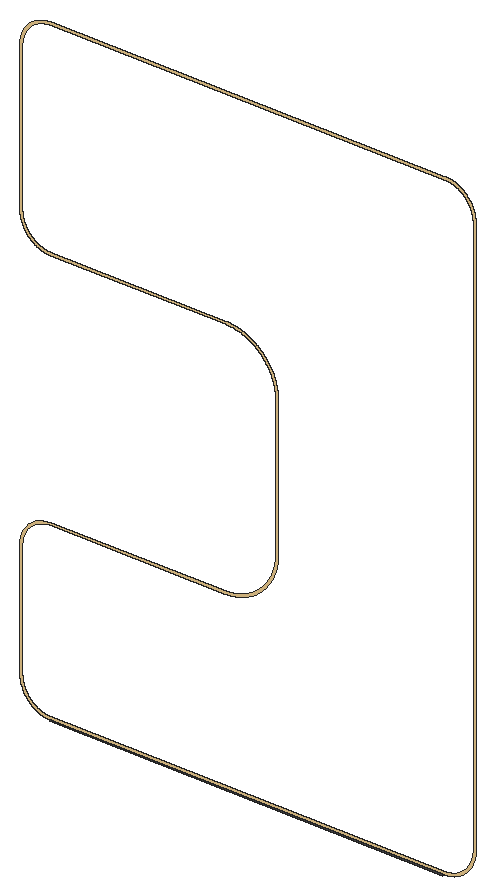
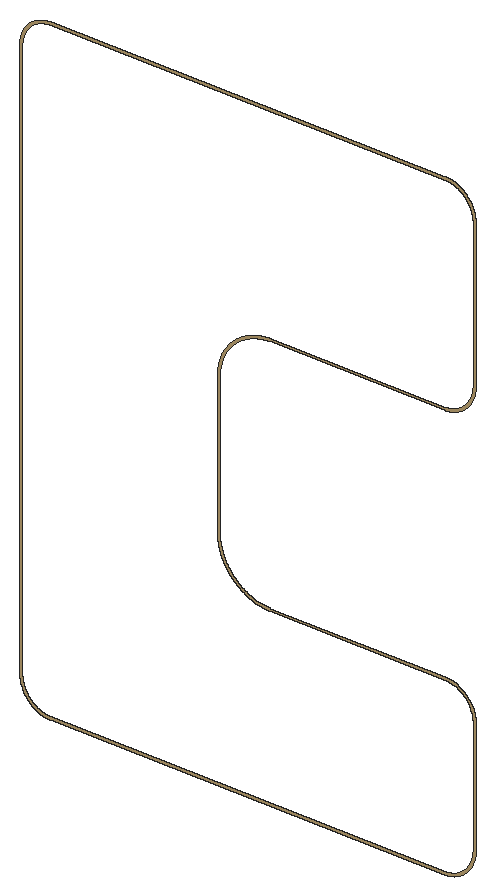
# SketchUp Ruby script. Lengths in inches.
U = 1.inch
M = Sketchup.active_model
def pt(a) = Geom::Point3d.new(a.map { |v| v * U })
def face(e, loops, mat)
  f = e.add_face(loops[0].map { |a| pt(a) })
  loops[1..].each { |l| e.add_face(l.map { |a| pt(a) }).erase! }
  f.material = f.back_material = mat if mat
  f
end
# faces: each face lists its corners as indices into pts; further lists are holes
def faces(e, pts, list, mat = nil) = list.each { |f| face(e, (f[0].is_a?(Array) ? f : [f]).map { |l| l.map { |i| pts[i] } }, mat) }
# xy, xz, yz: faces in a plane at the given z, y or x. An outline is a flat list of corners, or four numbers for a rectangle; further outlines are holes
def ring(l) = l.size == 4 ? [[l[0], l[1]], [l[2], l[1]], [l[2], l[3]], [l[0], l[3]]] : l.each_slice(2).to_a
def flat(e, list, mat, &to3) = list.each { |f| face(e, (f[0].is_a?(Array) ? f : [f]).map { |l| ring(l).map { |u, v| to3.(u, v) } }, mat) }
def xy(e, z, list, mat = nil) = flat(e, list, mat) { |x, y| [x, y, z] }
def xz(e, y, list, mat = nil) = flat(e, list, mat) { |x, z| [x, y, z] }
def yz(e, x, list, mat = nil) = flat(e, list, mat) { |y, z| [x, y, z] }
def lines(e, pts, list) = list.each { |a, b| e.add_line(pt(pts[a]), pt(pts[b])) }
# prism: a flat outline (further loops are holes) pulled along v
def prism(e, loops, v, mat = nil)
  f = face(e, loops, mat); d = Geom::Vector3d.new(v.map { |x| x * U })
  f.pushpull(f.normal.samedirection?(d) ? d.length : -d.length)
end
def box(e, o, s, mat = nil) = prism(e, [[o, [o[0] + s[0], o[1], o[2]], [o[0] + s[0], o[1] + s[1], o[2]], [o[0], o[1] + s[1], o[2]]]], [0, 0, s[2]], mat)
def at(x, y, z, deg = 0) = Geom::Transformation.translation(pt([x, y, z])) * Geom::Transformation.rotation(ORIGIN, Z_AXIS, deg.degrees)
def axes(o, x, y, z) = Geom::Transformation.new([*x, 0, *y, 0, *z, 0, *pt(o).to_a, 1])
def part(name) = M.definitions.add(name)
# library, detail: a bought-in or finely detailed component or shape, given as its bounding box
def library(name, o, s) = part(name).tap { |d| box(d.entities, o, s) }
def detail(e, o, s) = box(e.add_group.entities, o, s)
def put(e, d, t, mat = nil) = e.add_instance(d, t).tap { |i| i.material = mat if mat }
def group(e, t, mat = nil) = e.add_group.tap { |g| g.transformation = t; g.material = mat if mat }.entities
root = M.entities
M.materials.add("1432 AP 8245 TAR ROAD").color = [71, 72, 75]
M.materials.add("Outer Light").color = [251, 217, 152]
xy(root,171.29,[[279,95.37,537,96.87]],"1432 AP 8245 TAR ROAD")
xz(root,96.87,[[[278.68,171.29,278.52,171.3,278.36,171.3,278.2,171.31,278.03,171.31,277.875,171.32,277.71,171.33,277.55,171.34,277.39,171.36,277.07,171.38,276.75,171.42,276.59,171.43,276.27,171.47,276.11,171.5,275.79,171.54,275.63,171.57,275.48,171.6,275.32,171.625,275.16,171.66,275,171.6875,274.84,171.72,274.69,171.75,274.53,171.79,274.37,171.82,274.21,171.86,274.06,171.9,273.9,171.9375,273.75,171.98,273.59,172.02,273.44,172.0625,273.28,172.11,273.125,172.15,272.97,172.2,272.67,172.3,272.51,172.35,272.06,172.5,271.9,172.56,271.75,172.62,271.6,172.67,271.15,172.85,271.01,172.91,270.86,172.98,270.71,173.04,270.5625,173.11,270.42,173.18,270.27,173.24,270.125,173.3125,269.98,173.38,269.84,173.45,269.69,173.53,269.41,173.67,269.27,173.75,268.98,173.91,268.56,174.15,268.43,174.23,268.29,174.3125,268.15,174.4,268.02,174.48,267.88,174.57,267.75,174.66,267.61,174.75,267.48,174.84,267.34,174.93,267.08,175.11,266.95,175.21,266.82,175.3,266.69,175.4,266.5625,175.5,266.44,175.59,266.18,175.79,266.06,175.89,265.93,176,265.81,176.1,265.6875,176.2,265.5625,176.31,265.44,176.41,265.08,176.74,264.97,176.85,264.73,177.07,264.39,177.41,264.28,177.53,264.17,177.64,264.06,177.76,263.95,177.875,263.84,178,263.73,178.11,263.62,178.24,263.52,178.36,263.41,178.48,263.31,178.6,263.2,178.72,263.1,178.85,263,178.97,262.7,179.36,262.61,179.48,262.51,179.61,262.42,179.74,262.32,179.875,262.23,180,262.14,180.14,262.04,180.27,261.95,180.4,261.87,180.54,261.78,180.67,261.69,180.81,261.61,180.94,261.52,181.08,261.4375,181.22,261.35,181.36,261.11,181.78,261.04,181.92,260.88,182.2,260.81,182.34,260.73,182.49,260.59,182.77,260.52,182.92,260.45,183.0625,260.38,183.21,260.32,183.36,260.25,183.5,260.1875,183.65,260.12,183.8,259.82,184.55,259.77,184.7,259.71,184.85,259.61,185.15,259.55,185.3,259.5,185.46,259.45,185.61,259.41,185.76,259.36,185.92,259.3125,186.07,259.27,186.23,259.23,186.38,259.18,186.54,259.14,186.69,259.1,186.85,259.07,187.01,259.03,187.16,258.99,187.32,258.96,187.48,258.93,187.63,258.89,187.79,258.83,188.11,258.81,188.27,258.75,188.59,258.73,188.74,258.7,188.9,258.68,189.0625,258.66,189.22,258.64,189.38,258.61,189.7,258.59,189.86,258.58,190.02,258.5625,190.18,258.55,190.34,258.54,190.5,258.53,190.67,258.52,190.83,258.52,190.99,258.51,191.15,258.51,191.31,258.5,191.47,258.5,266.79,258.68,269.47,259.2,272.1,260.06,274.64,261.25,277.04,262.74,279.27,264.5,281.29,266.52,283.06,268.75,284.55,271.15,285.73,273.69,286.59,276.32,287.12,279,287.29,393.4375,287.29,393.875,287.3,394.32,287.32,394.75,287.34,395.19,287.36,395.63,287.4,396.07,287.43,396.5,287.48,396.9375,287.52,397.37,287.58,397.81,287.64,398.24,287.7,398.67,287.78,399.1,287.85,399.54,287.9375,399.97,288.02,400.39,288.12,401.25,288.32,401.67,288.43,402.51,288.67,403.35,288.93,403.77,289.07,404.18,289.21,404.59,289.36,405.01,289.52,405.41,289.68,405.82,289.84,406.22,290.01,406.625,290.1875,407.03,290.37,407.42,290.56,407.82,290.75,408.21,290.94,408.6,291.14,408.98,291.35,409.37,291.5625,409.75,291.78,410.13,292,410.5,292.23,410.875,292.46,411.25,292.7,411.61,292.9375,411.97,293.18,412.33,293.43,412.69,293.69,413.39,294.21,413.74,294.48,414.76,295.32,415.42,295.9,415.74,296.19,416.06,296.49,416.375,296.8,416.6875,297.1,417,297.42,417.3,297.73,417.6,298.05,417.9,298.375,418.1875,298.7,418.47,299.04,418.76,299.37,419.03,299.71,419.31,300.05,419.58,300.4,420.1,301.1,420.36,301.46,420.61,301.82,420.85,302.18,421.1,302.55,421.33,302.92,421.5625,303.29,421.79,303.66,422.23,304.42,422.44,304.81,422.65,305.19,422.85,305.58,423.05,305.98,423.24,306.37,423.78,307.57,423.95,307.97,424.12,308.38,424.27,308.79,424.43,309.2,424.58,309.61,424.72,310.02,424.86,310.44,425.12,311.28,425.36,312.12,425.47,312.55,425.57,312.97,425.77,313.83,425.86,314.26,425.9375,314.6875,426.02,315.12,426.09,315.55,426.15,315.99,426.27,316.85,426.32,317.29,426.36,317.73,426.4,318.16,426.43,318.6,426.49,319.92,426.5,320.35,426.5,411.23,426.49,411.67,426.45,412.55,426.43,412.98,426.4,413.42,426.36,413.86,426.32,414.29,426.27,414.73,426.21,415.16,426.15,415.6,426.09,416.03,426.02,416.47,425.9375,416.9,425.86,417.33,425.77,417.76,425.67,418.19,425.57,418.61,425.47,419.04,425.36,419.46,425.24,419.89,425.12,420.31,424.99,420.73,424.86,421.14,424.72,421.56,424.58,421.97,424.43,422.39,424.27,422.8,424.12,423.21,423.95,423.61,423.78,424.02,423.42,424.82,423.24,425.21,423.05,425.61,422.65,426.39,422.44,426.78,422.23,427.16,421.79,427.92,421.5625,428.3,421.33,428.67,421.1,429.04,420.85,429.4,420.61,429.77,420.36,430.125,420.1,430.48,419.84,430.84,419.58,431.1875,419.31,431.53,419.03,431.875,418.76,432.21,418.47,432.55,418.1875,432.88,417.9,433.21,417,434.17,416.375,434.79,416.06,435.09,415.74,435.39,415.42,435.6875,415.09,435.98,414.76,436.27,414.08,436.83,413.74,437.1,413.39,437.37,412.69,437.89,412.33,438.15,411.61,438.65,411.25,438.89,410.5,439.36,410.13,439.58,409.37,440.02,408.98,440.23,408.6,440.4375,408.21,440.64,407.82,440.84,407.42,441.03,407.03,441.21,406.625,441.4,406.22,441.57,405.82,441.74,405.41,441.91,405.01,442.07,404.59,442.22,404.18,442.37,403.77,442.51,402.93,442.79,401.67,443.15,401.25,443.26,400.82,443.37,400.39,443.47,399.97,443.56,399.54,443.65,399.1,443.73,398.67,443.81,397.81,443.95,397.37,444.01,396.9375,444.06,396.5,444.11,396.07,444.15,395.63,444.1875,395.19,444.22,394.75,444.25,394.32,444.27,393.875,444.28,393.4375,444.29,278.68,444.29,278.52,444.3,278.36,444.3,278.2,444.31,278.03,444.31,277.875,444.32,277.71,444.33,277.55,444.34,277.39,444.36,277.07,444.38,276.75,444.42,276.59,444.43,276.27,444.47,276.11,444.5,275.79,444.54,275.63,444.57,275.48,444.6,275.32,444.625,275.16,444.66,275,444.6875,274.84,444.72,274.69,444.75,274.53,444.79,274.37,444.82,274.21,444.86,274.06,444.9,273.9,444.9375,273.75,444.98,273.59,445.02,273.44,445.0625,273.28,445.11,273.125,445.15,272.97,445.2,272.67,445.3,272.51,445.35,272.06,445.5,271.9,445.56,271.75,445.62,271.6,445.67,271.15,445.85,271.01,445.91,270.86,445.98,270.71,446.04,270.5625,446.11,270.42,446.18,270.27,446.24,270.125,446.3125,269.98,446.38,269.84,446.45,269.69,446.53,269.41,446.67,269.27,446.75,268.98,446.91,268.56,447.15,268.43,447.23,268.29,447.3125,268.15,447.4,268.02,447.48,267.88,447.57,267.75,447.66,267.61,447.75,267.48,447.84,267.34,447.93,267.08,448.11,266.95,448.21,266.82,448.3,266.69,448.4,266.5625,448.5,266.44,448.59,266.18,448.79,266.06,448.89,265.93,449,265.81,449.1,265.6875,449.2,265.5625,449.31,265.44,449.41,265.08,449.74,264.97,449.85,264.73,450.07,264.39,450.41,264.28,450.53,264.17,450.64,264.06,450.76,263.95,450.875,263.84,451,263.73,451.11,263.62,451.24,263.52,451.36,263.41,451.48,263.31,451.6,263.2,451.72,263.1,451.85,263,451.97,262.7,452.36,262.61,452.48,262.51,452.61,262.42,452.74,262.32,452.875,262.23,453,262.14,453.14,262.04,453.27,261.95,453.4,261.87,453.54,261.78,453.67,261.69,453.81,261.61,453.94,261.52,454.08,261.4375,454.22,261.35,454.36,261.11,454.78,261.04,454.92,260.88,455.2,260.81,455.34,260.73,455.49,260.59,455.77,260.52,455.92,260.45,456.0625,260.38,456.21,260.32,456.36,260.25,456.5,260.1875,456.65,260.12,456.8,259.82,457.55,259.77,457.7,259.71,457.85,259.61,458.15,259.55,458.3,259.5,458.46,259.45,458.61,259.41,458.76,259.36,458.92,259.3125,459.07,259.27,459.23,259.23,459.38,259.18,459.54,259.14,459.69,259.1,459.85,259.07,460.01,259.03,460.16,258.99,460.32,258.96,460.48,258.93,460.63,258.89,460.79,258.83,461.11,258.81,461.27,258.75,461.59,258.73,461.74,258.7,461.9,258.68,462.0625,258.66,462.22,258.64,462.38,258.61,462.7,258.59,462.86,258.58,463.02,258.5625,463.18,258.55,463.34,258.54,463.5,258.53,463.67,258.52,463.83,258.52,463.99,258.51,464.15,258.51,464.31,258.5,464.47,258.5,561.11,258.51,561.28,258.51,561.4375,258.52,561.6,258.52,561.76,258.55,562.24,258.5625,562.4,258.58,562.5625,258.59,562.72,258.61,562.88,258.64,563.2,258.7,563.68,258.73,563.84,258.75,564,258.81,564.32,258.83,564.48,258.86,564.63,258.89,564.79,258.93,564.95,258.96,565.11,258.99,565.26,259.07,565.58,259.1,565.73,259.18,566.05,259.23,566.2,259.27,566.36,259.3125,566.51,259.36,566.67,259.41,566.82,259.45,566.97,259.55,567.28,259.61,567.43,259.66,567.58,259.71,567.74,259.77,567.89,259.82,568.04,259.88,568.1875,259.94,568.34,260.12,568.79,260.1875,568.93,260.25,569.08,260.32,569.23,260.38,569.375,260.45,569.52,260.52,569.67,260.59,569.8125,260.66,569.96,260.73,570.1,260.81,570.24,260.88,570.38,260.96,570.53,261.04,570.67,261.11,570.81,261.35,571.23,261.4375,571.37,261.52,571.5,261.61,571.64,261.69,571.78,261.78,571.91,261.87,572.05,261.95,572.18,262.04,572.31,262.14,572.45,262.32,572.71,262.42,572.84,262.51,572.97,262.61,573.1,262.7,573.23,262.8,573.36,262.9,573.48,263,573.61,263.1,573.73,263.2,573.86,263.31,573.98,263.41,574.11,263.52,574.23,263.62,574.35,264.06,574.83,264.17,574.94,264.28,575.06,264.39,575.17,264.5,575.29,264.62,575.4,264.73,575.51,264.97,575.74,265.08,575.85,265.2,575.95,265.32,576.0625,265.44,576.17,265.5625,576.28,265.6875,576.38,265.81,576.48,265.93,576.59,266.06,576.69,266.18,576.79,266.44,576.99,266.5625,577.09,266.69,577.1875,266.82,577.28,267.08,577.47,267.21,577.5625,267.34,577.66,267.48,577.75,267.61,577.84,267.75,577.93,267.88,578.01,268.02,578.1,268.15,578.1875,268.29,578.27,268.43,578.35,268.56,578.4375,268.7,578.52,268.98,578.68,269.125,578.76,269.27,578.83,269.41,578.91,269.55,578.98,269.69,579.06,269.84,579.13,269.98,579.2,270.27,579.34,270.42,579.41,270.5625,579.48,270.71,579.54,270.86,579.61,271.01,579.67,271.15,579.73,271.75,579.97,271.9,580.02,272.06,580.08,272.21,580.13,272.36,580.1875,272.51,580.24,272.67,580.29,272.97,580.39,273.125,580.43,273.28,580.48,273.44,580.52,273.59,580.57,273.75,580.61,273.9,580.65,274.06,580.6875,274.21,580.73,274.37,580.76,274.53,580.8,274.69,580.83,274.84,580.87,275.48,580.99,275.63,581.01,275.79,581.04,275.95,581.0625,276.11,581.09,276.91,581.19,277.07,581.2,277.23,581.22,277.71,581.25,277.875,581.26,278.03,581.27,278.2,581.28,278.36,581.28,278.52,581.29,537.48,581.29,537.64,581.28,537.8,581.28,537.97,581.27,538.125,581.26,538.29,581.25,538.77,581.22,538.93,581.2,539.09,581.19,539.89,581.09,540.05,581.0625,540.21,581.04,540.37,581.01,540.52,580.99,541.16,580.87,541.31,580.83,541.47,580.8,541.63,580.76,541.79,580.73,541.94,580.6875,542.1,580.65,542.25,580.61,542.41,580.57,542.56,580.52,542.72,580.48,542.875,580.43,543.03,580.39,543.33,580.29,543.49,580.24,543.64,580.1875,543.79,580.13,543.94,580.08,544.1,580.02,544.25,579.97,544.85,579.73,544.99,579.67,545.14,579.61,545.29,579.54,545.4375,579.48,545.58,579.41,545.73,579.34,546.02,579.2,546.16,579.13,546.31,579.06,546.45,578.98,546.59,578.91,546.73,578.83,546.875,578.76,547.02,578.68,547.3,578.52,547.44,578.4375,547.57,578.35,547.71,578.27,547.85,578.1875,547.98,578.1,548.12,578.01,548.25,577.93,548.39,577.84,548.52,577.75,548.66,577.66,548.79,577.5625,548.92,577.47,549.18,577.28,549.31,577.1875,549.4375,577.09,549.56,576.99,549.82,576.79,549.94,576.69,550.07,576.59,550.19,576.48,550.3125,576.38,550.4375,576.28,550.56,576.17,550.68,576.0625,550.8,575.95,550.92,575.85,551.03,575.74,551.27,575.51,551.38,575.4,551.5,575.29,551.61,575.17,551.72,575.06,551.83,574.94,551.94,574.83,552.38,574.35,552.48,574.23,552.59,574.11,552.69,573.98,552.8,573.86,552.9,573.73,553,573.61,553.1,573.48,553.2,573.36,553.3,573.23,553.39,573.1,553.49,572.97,553.58,572.84,553.68,572.71,553.86,572.45,553.96,572.31,554.05,572.18,554.13,572.05,554.22,571.91,554.31,571.78,554.39,571.64,554.48,571.5,554.5625,571.37,554.65,571.23,554.89,570.81,554.96,570.67,555.04,570.53,555.12,570.38,555.19,570.24,555.27,570.1,555.34,569.96,555.41,569.8125,555.48,569.67,555.55,569.52,555.62,569.375,555.68,569.23,555.75,569.08,555.8125,568.93,555.88,568.79,556.06,568.34,556.12,568.1875,556.18,568.04,556.23,567.89,556.29,567.74,556.34,567.58,556.39,567.43,556.45,567.28,556.55,566.97,556.59,566.82,556.64,566.67,556.6875,566.51,556.73,566.36,556.77,566.2,556.82,566.05,556.9,565.73,556.93,565.58,557.01,565.26,557.04,565.11,557.07,564.95,557.11,564.79,557.14,564.63,557.17,564.48,557.19,564.32,557.25,564,557.27,563.84,557.3,563.68,557.36,563.2,557.39,562.88,557.41,562.72,557.42,562.5625,557.4375,562.4,557.45,562.24,557.48,561.76,557.48,561.6,557.49,561.4375,557.49,561.28,557.5,561.11,557.5,191.47,557.49,191.31,557.49,191.15,557.48,190.99,557.48,190.83,557.47,190.67,557.46,190.5,557.45,190.34,557.4375,190.18,557.42,190.02,557.41,189.86,557.39,189.7,557.36,189.38,557.34,189.22,557.32,189.0625,557.3,188.9,557.27,188.74,557.25,188.59,557.19,188.27,557.17,188.11,557.11,187.79,557.07,187.63,557.04,187.48,557.01,187.32,556.97,187.16,556.93,187.01,556.9,186.85,556.86,186.69,556.82,186.54,556.77,186.38,556.73,186.23,556.6875,186.07,556.64,185.92,556.59,185.76,556.55,185.61,556.5,185.46,556.45,185.3,556.39,185.15,556.29,184.85,556.23,184.7,556.18,184.55,555.88,183.8,555.8125,183.65,555.75,183.5,555.68,183.36,555.62,183.21,555.55,183.0625,555.48,182.92,555.41,182.77,555.27,182.49,555.19,182.34,555.12,182.2,554.96,181.92,554.89,181.78,554.65,181.36,554.5625,181.22,554.48,181.08,554.39,180.94,554.31,180.81,554.22,180.67,554.13,180.54,554.05,180.4,553.96,180.27,553.86,180.14,553.77,180,553.68,179.875,553.58,179.74,553.49,179.61,553.39,179.48,553.3,179.36,553,178.97,552.9,178.85,552.8,178.72,552.69,178.6,552.59,178.48,552.48,178.36,552.38,178.24,552.27,178.11,552.16,178,552.05,177.875,551.94,177.76,551.83,177.64,551.72,177.53,551.61,177.41,551.27,177.07,551.03,176.85,550.92,176.74,550.56,176.41,550.4375,176.31,550.3125,176.2,550.19,176.1,550.07,176,549.94,175.89,549.82,175.79,549.56,175.59,549.4375,175.5,549.31,175.4,549.18,175.3,549.05,175.21,548.92,175.11,548.66,174.93,548.52,174.84,548.39,174.75,548.25,174.66,548.12,174.57,547.98,174.48,547.85,174.4,547.71,174.3125,547.57,174.23,547.44,174.15,547.02,173.91,546.73,173.75,546.59,173.67,546.31,173.53,546.16,173.45,546.02,173.38,545.875,173.3125,545.73,173.24,545.58,173.18,545.4375,173.11,545.29,173.04,545.14,172.98,544.99,172.91,544.85,172.85,544.4,172.67,544.25,172.62,544.1,172.56,543.94,172.5,543.49,172.35,543.33,172.3,543.03,172.2,542.875,172.15,542.72,172.11,542.56,172.0625,542.41,172.02,542.25,171.98,542.1,171.9375,541.94,171.9,541.79,171.86,541.63,171.82,541.47,171.79,541.31,171.75,541.16,171.72,541,171.6875,540.84,171.66,540.68,171.625,540.52,171.6,540.37,171.57,540.21,171.54,539.89,171.5,539.73,171.47,539.41,171.43,539.25,171.42,538.93,171.38,538.61,171.36,538.45,171.34,538.29,171.33,538.125,171.32,537.97,171.31,537.8,171.31,537.64,171.3,537.48,171.3,537.32,171.29],[278.7,172.79,537.3,172.79,537.45,172.8,537.6,172.8,537.75,172.81,537.9,172.8125,538.04,172.82,538.64,172.86,538.79,172.875,538.9375,172.89,539.08,172.91,539.23,172.92,539.68,172.98,539.82,173,539.97,173.03,540.27,173.07,540.41,173.1,540.71,173.16,540.85,173.1875,541,173.22,541.14,173.25,541.29,173.28,541.44,173.32,541.58,173.35,541.73,173.39,542.01,173.47,542.16,173.51,542.44,173.59,542.59,173.63,542.73,173.68,542.87,173.72,543.15,173.82,543.3,173.87,543.4375,173.92,543.58,173.97,543.86,174.07,543.99,174.125,544.13,174.18,544.41,174.3,544.55,174.35,544.68,174.41,544.82,174.48,544.95,174.54,545.09,174.6,545.22,174.66,545.36,174.73,545.49,174.8,545.625,174.86,545.76,174.93,546.28,175.21,546.41,175.29,546.54,175.36,546.67,175.4375,546.8,175.51,546.93,175.59,547.05,175.67,547.31,175.83,547.43,175.91,547.56,175.99,547.68,176.08,547.8,176.16,547.93,176.25,548.05,176.33,548.41,176.6,548.53,176.6875,548.65,176.78,548.76,176.87,548.88,176.96,549,177.06,549.11,177.15,549.23,177.25,549.34,177.34,549.56,177.54,549.68,177.64,550.01,177.94,550.22,178.15,550.33,178.25,550.54,178.46,550.64,178.57,550.75,178.68,550.85,178.79,550.95,178.89,551.05,179,551.15,179.12,551.45,179.45,551.54,179.57,551.64,179.68,551.73,179.8,551.83,179.91,552.1,180.27,552.19,180.38,552.28,180.5,552.46,180.75,552.54,180.87,552.63,180.99,552.71,181.11,552.8,181.24,552.88,181.36,552.96,181.49,553.04,181.61,553.12,181.74,553.2,181.86,553.28,181.99,553.35,182.12,553.43,182.25,553.5,182.38,553.58,182.51,553.86,183.03,553.93,183.17,554,183.3,554.0625,183.43,554.13,183.57,554.19,183.7,554.25,183.84,554.32,183.97,554.38,184.11,554.4375,184.25,554.5,184.38,554.55,184.52,554.67,184.8,554.72,184.9375,554.77,185.08,554.83,185.22,554.875,185.36,554.93,185.5,554.98,185.64,555.02,185.78,555.07,185.92,555.12,186.0625,555.16,186.21,555.2,186.35,555.25,186.49,555.29,186.63,555.33,186.78,555.37,186.92,555.4,187.07,555.44,187.21,555.48,187.36,555.51,187.5,555.54,187.65,555.57,187.79,555.61,187.9375,555.63,188.09,555.66,188.23,555.72,188.53,555.74,188.67,555.77,188.82,555.79,188.97,555.81,189.11,555.89,189.71,555.9,189.86,555.92,190,555.99,191.05,555.99,191.34,556,191.49,556,561.09,555.99,561.24,555.99,561.54,555.98,561.6875,555.97,561.84,555.96,561.99,555.95,562.13,555.92,562.58,555.9,562.73,555.89,562.88,555.87,563.03,555.85,563.17,555.79,563.62,555.77,563.76,555.74,563.91,555.72,564.06,555.69,564.21,555.66,564.35,555.63,564.5,555.61,564.65,555.57,564.79,555.54,564.9375,555.51,565.08,555.48,565.23,555.44,565.37,555.4,565.52,555.37,565.66,555.33,565.81,555.25,566.09,555.2,566.24,555.12,566.52,555.07,566.66,555.02,566.81,554.98,566.95,554.93,567.09,554.875,567.23,554.83,567.37,554.77,567.51,554.67,567.79,554.61,567.92,554.55,568.0625,554.5,568.2,554.4375,568.34,554.38,568.47,554.32,568.61,554.25,568.75,554.19,568.88,554.13,569.02,554.0625,569.15,554,569.28,553.93,569.42,553.79,569.68,553.72,569.8125,553.65,569.95,553.58,570.08,553.5,570.21,553.43,570.34,553.35,570.46,553.28,570.59,553.12,570.85,553.04,570.97,552.96,571.1,552.88,571.22,552.8,571.35,552.71,571.47,552.63,571.59,552.54,571.72,552.46,571.84,552.1,572.32,552.01,572.4375,551.92,572.55,551.83,572.67,551.73,572.79,551.64,572.9,551.54,573.02,551.45,573.13,551.35,573.24,551.25,573.36,551.05,573.58,550.95,573.6875,550.85,573.8,550.75,573.91,550.64,574.01,550.44,574.23,550.33,574.33,550.22,574.4375,550.11,574.54,550.01,574.64,549.9,574.74,549.79,574.85,549.68,574.95,549.56,575.04,549.23,575.34,549.11,575.43,549,575.53,548.76,575.71,548.65,575.8,548.53,575.9,548.29,576.08,548.17,576.16,547.93,576.34,547.8,576.42,547.68,576.51,547.56,576.59,547.43,576.67,547.31,576.75,547.05,576.91,546.93,576.99,546.67,577.15,546.54,577.22,546.41,577.3,545.76,577.65,545.49,577.79,545.36,577.85,545.22,577.92,545.09,577.98,544.95,578.05,544.82,578.11,544.68,578.17,544.55,578.23,544.27,578.35,544.13,578.4,543.99,578.46,543.86,578.51,543.72,578.57,543.58,578.62,543.4375,578.67,543.3,578.72,543.15,578.77,543.01,578.82,542.87,578.86,542.73,578.91,542.59,578.95,542.44,579,542.16,579.08,542.01,579.12,541.73,579.2,541.58,579.23,541.44,579.27,541.14,579.33,541,579.37,540.85,579.4,540.71,579.43,540.56,579.46,540.41,579.48,540.27,579.51,540.12,579.53,539.97,579.56,539.82,579.58,539.68,579.6,539.08,579.68,538.9375,579.69,538.79,579.71,538.04,579.76,537.9,579.77,537.75,579.78,537.6,579.78,537.45,579.79,278.55,579.79,278.4,579.78,278.25,579.78,278.1,579.77,277.96,579.76,277.21,579.71,277.0625,579.69,276.92,579.68,276.32,579.6,276.18,579.58,276.03,579.56,275.88,579.53,275.73,579.51,275.59,579.48,275.44,579.46,275.29,579.43,275.15,579.4,275,579.37,274.86,579.33,274.56,579.27,274.42,579.23,274.27,579.2,273.99,579.12,273.84,579.08,273.56,579,273.41,578.95,273.27,578.91,273.13,578.86,272.99,578.82,272.85,578.77,272.7,578.72,272.5625,578.67,272.42,578.62,272.28,578.57,272.14,578.51,272.01,578.46,271.87,578.4,271.73,578.35,271.45,578.23,271.32,578.17,271.18,578.11,271.05,578.05,270.91,577.98,270.78,577.92,270.64,577.85,270.51,577.79,270.24,577.65,269.59,577.3,269.46,577.22,269.33,577.15,269.07,576.99,268.95,576.91,268.69,576.75,268.57,576.67,268.44,576.59,268.32,576.51,268.2,576.42,268.07,576.34,267.83,576.16,267.71,576.08,267.47,575.9,267.35,575.8,267.24,575.71,267,575.53,266.89,575.43,266.77,575.34,266.44,575.04,266.32,574.95,266.21,574.85,266.1,574.74,265.99,574.64,265.89,574.54,265.78,574.4375,265.67,574.33,265.56,574.23,265.36,574.01,265.25,573.91,265.15,573.8,265.05,573.6875,264.95,573.58,264.75,573.36,264.65,573.24,264.55,573.13,264.46,573.02,264.36,572.9,264.27,572.79,264.17,572.67,264.08,572.55,263.99,572.4375,263.9,572.32,263.54,571.84,263.46,571.72,263.37,571.59,263.29,571.47,263.2,571.35,263.12,571.22,263.04,571.1,262.96,570.97,262.88,570.85,262.72,570.59,262.65,570.46,262.57,570.34,262.5,570.21,262.42,570.08,262.35,569.95,262.28,569.8125,262.21,569.68,262.07,569.42,262,569.28,261.9375,569.15,261.87,569.02,261.81,568.88,261.75,568.75,261.68,568.61,261.62,568.47,261.5625,568.34,261.5,568.2,261.45,568.0625,261.39,567.92,261.33,567.79,261.23,567.51,261.17,567.37,261.125,567.23,261.07,567.09,261.02,566.95,260.98,566.81,260.93,566.66,260.88,566.52,260.8,566.24,260.75,566.09,260.67,565.81,260.63,565.66,260.6,565.52,260.56,565.37,260.52,565.23,260.49,565.08,260.46,564.9375,260.43,564.79,260.39,564.65,260.37,564.5,260.34,564.35,260.31,564.21,260.28,564.06,260.26,563.91,260.23,563.76,260.21,563.62,260.15,563.17,260.13,563.03,260.11,562.88,260.1,562.73,260.08,562.58,260.05,562.13,260.04,561.99,260.03,561.84,260.02,561.6875,260.01,561.54,260.01,561.24,260,561.09,260,464.49,260.01,464.34,260.01,464.05,260.08,463,260.1,462.86,260.11,462.71,260.19,462.11,260.21,461.97,260.23,461.82,260.26,461.67,260.28,461.53,260.34,461.23,260.37,461.09,260.39,460.9375,260.43,460.79,260.46,460.65,260.49,460.5,260.52,460.36,260.56,460.21,260.6,460.07,260.63,459.92,260.67,459.78,260.71,459.63,260.75,459.49,260.8,459.35,260.84,459.21,260.88,459.0625,260.93,458.92,260.98,458.78,261.02,458.64,261.07,458.5,261.125,458.36,261.17,458.22,261.23,458.08,261.28,457.9375,261.33,457.8,261.45,457.52,261.5,457.38,261.5625,457.25,261.62,457.11,261.68,456.97,261.75,456.84,261.81,456.7,261.87,456.57,261.9375,456.43,262,456.3,262.07,456.17,262.14,456.03,262.42,455.51,262.5,455.38,262.57,455.25,262.65,455.12,262.72,454.99,262.8,454.86,262.88,454.74,262.96,454.61,263.04,454.49,263.12,454.36,263.2,454.24,263.29,454.11,263.37,453.99,263.46,453.87,263.54,453.75,263.72,453.5,263.81,453.38,263.9,453.27,264.17,452.91,264.27,452.8,264.36,452.68,264.46,452.57,264.55,452.45,264.85,452.12,264.95,452,265.05,451.89,265.15,451.79,265.25,451.68,265.36,451.57,265.46,451.46,265.67,451.25,265.78,451.15,265.99,450.94,266.32,450.64,266.44,450.54,266.66,450.34,266.77,450.25,266.89,450.15,267,450.06,267.12,449.96,267.24,449.87,267.35,449.78,267.47,449.6875,267.59,449.6,267.95,449.33,268.07,449.25,268.2,449.16,268.32,449.08,268.44,448.99,268.57,448.91,268.69,448.83,268.95,448.67,269.07,448.59,269.2,448.51,269.33,448.4375,269.46,448.36,269.59,448.29,269.72,448.21,270.24,447.93,270.375,447.86,270.51,447.8,270.64,447.73,270.78,447.66,270.91,447.6,271.05,447.54,271.18,447.48,271.32,447.41,271.45,447.35,271.59,447.3,271.87,447.18,272.01,447.125,272.14,447.07,272.42,446.97,272.5625,446.92,272.7,446.87,272.85,446.82,273.13,446.72,273.27,446.68,273.41,446.63,273.56,446.59,273.84,446.51,273.99,446.47,274.27,446.39,274.42,446.35,274.56,446.32,274.71,446.28,274.86,446.25,275,446.22,275.15,446.1875,275.29,446.16,275.59,446.1,275.73,446.07,276.03,446.03,276.18,446,276.32,445.98,276.77,445.92,276.92,445.91,277.0625,445.89,277.21,445.875,277.36,445.86,277.96,445.82,278.1,445.8125,278.25,445.81,278.4,445.8,278.55,445.8,278.7,445.79,393.46,445.79,393.92,445.78,394.375,445.77,394.83,445.74,395.29,445.72,395.75,445.68,396.2,445.65,396.66,445.6,397.11,445.55,397.57,445.49,398.02,445.43,398.48,445.36,398.93,445.29,399.38,445.21,400.28,445.03,400.72,444.93,401.17,444.82,401.62,444.72,402.5,444.48,403.38,444.22,403.82,444.08,405.11,443.63,405.54,443.47,405.97,443.3,406.39,443.13,406.82,442.95,407.24,442.77,407.65,442.58,408.07,442.38,408.89,441.98,409.3,441.77,410.1,441.33,410.9,440.87,411.68,440.39,412.0625,440.15,412.44,439.89,412.82,439.64,413.2,439.375,413.57,439.11,413.94,438.84,414.31,438.56,414.67,438.28,415.03,437.99,415.73,437.41,416.08,437.11,416.76,436.49,417.09,436.18,417.75,435.54,418.39,434.88,418.7,434.55,419.01,434.21,419.3125,433.87,419.61,433.52,419.91,433.17,420.2,432.82,420.49,432.46,420.77,432.1,421.04,431.73,421.32,431.36,421.84,430.62,422.1,430.24,422.35,429.85,422.6,429.47,422.84,429.08,423.08,428.6875,423.3125,428.29,423.54,427.89,423.76,427.49,423.97,427.09,424.19,426.68,424.79,425.45,424.97,425.03,425.16,424.61,425.34,424.1875,425.51,423.76,425.68,423.33,425.84,422.91,425.99,422.48,426.14,422.04,426.29,421.61,426.43,421.17,426.56,420.73,426.6875,420.29,426.81,419.85,426.92,419.41,427.03,418.96,427.14,418.52,427.24,418.07,427.33,417.62,427.57,416.27,427.64,415.8125,427.7,415.36,427.76,414.91,427.81,414.45,427.85,413.99,427.89,413.54,427.93,413.08,427.97,412.17,427.99,411.71,428,411.25,428,320.33,427.99,319.875,427.97,319.42,427.93,318.5,427.89,318.05,427.81,317.13,427.76,316.68,427.7,316.22,427.64,315.77,427.57,315.32,427.49,314.86,427.33,313.96,427.24,313.52,427.14,313.07,427.03,312.62,426.92,312.18,426.81,311.73,426.6875,311.29,426.56,310.85,426.43,310.41,426.29,309.98,426.14,309.54,425.84,308.68,425.68,308.25,425.51,307.82,425.34,307.4,425.16,306.98,424.97,306.56,424.79,306.14,424.59,305.72,424.39,305.3125,424.19,304.9,423.97,304.5,423.76,304.09,423.54,303.69,423.3125,303.29,423.08,302.9,422.84,302.5,422.6,302.12,422.35,301.73,422.1,301.35,421.58,300.59,421.32,300.22,421.04,299.85,420.77,299.49,420.49,299.125,420.2,298.77,419.91,298.41,419.61,298.0625,419.3125,297.71,419.01,297.37,418.7,297.03,418.39,296.7,417.75,296.04,417.09,295.4,416.76,295.09,416.42,294.78,416.08,294.48,415.38,293.88,415.03,293.59,414.67,293.31,414.31,293.02,413.2,292.21,412.44,291.69,412.0625,291.4375,411.68,291.19,410.9,290.71,410.1,290.25,409.7,290.03,409.3,289.82,408.48,289.4,408.07,289.2,407.65,289.01,407.24,288.82,406.82,288.63,406.39,288.46,405.97,288.28,404.68,287.8,404.25,287.65,403.82,287.51,402.94,287.23,402.5,287.11,402.06,286.98,401.62,286.87,401.17,286.76,400.72,286.66,400.28,286.56,399.83,286.46,398.48,286.22,398.02,286.15,397.57,286.09,397.11,286.03,396.66,285.98,396.2,285.9375,395.75,285.9,394.83,285.84,393.92,285.8,393.46,285.8,393,285.79,279,285.79,276.52,285.63,274.08,285.14,271.73,284.35,269.5,283.25,267.43,281.87,265.56,280.23,263.93,278.36,262.55,276.29,261.45,274.0625,260.65,271.71,260.16,269.27,260,266.79,260,191.49,260.01,191.34,260.01,191.05,260.08,190,260.1,189.86,260.11,189.71,260.19,189.11,260.21,188.97,260.23,188.82,260.26,188.67,260.28,188.53,260.34,188.23,260.37,188.09,260.39,187.9375,260.43,187.79,260.46,187.65,260.49,187.5,260.52,187.36,260.56,187.21,260.6,187.07,260.63,186.92,260.67,186.78,260.71,186.63,260.75,186.49,260.8,186.35,260.84,186.21,260.88,186.0625,260.93,185.92,260.98,185.78,261.02,185.64,261.07,185.5,261.125,185.36,261.17,185.22,261.23,185.08,261.28,184.9375,261.33,184.8,261.45,184.52,261.5,184.38,261.5625,184.25,261.62,184.11,261.68,183.97,261.75,183.84,261.81,183.7,261.87,183.57,261.9375,183.43,262,183.3,262.07,183.17,262.14,183.03,262.42,182.51,262.5,182.38,262.57,182.25,262.65,182.12,262.72,181.99,262.8,181.86,262.88,181.74,262.96,181.61,263.04,181.49,263.12,181.36,263.2,181.24,263.29,181.11,263.37,180.99,263.46,180.87,263.54,180.75,263.72,180.5,263.81,180.38,263.9,180.27,264.17,179.91,264.27,179.8,264.36,179.68,264.46,179.57,264.55,179.45,264.85,179.12,264.95,179,265.05,178.89,265.15,178.79,265.25,178.68,265.36,178.57,265.46,178.46,265.67,178.25,265.78,178.15,265.99,177.94,266.32,177.64,266.44,177.54,266.66,177.34,266.77,177.25,266.89,177.15,267,177.06,267.12,176.96,267.24,176.87,267.35,176.78,267.47,176.6875,267.59,176.6,267.95,176.33,268.07,176.25,268.2,176.16,268.32,176.08,268.44,175.99,268.57,175.91,268.69,175.83,268.95,175.67,269.07,175.59,269.2,175.51,269.33,175.4375,269.46,175.36,269.59,175.29,269.72,175.21,270.24,174.93,270.375,174.86,270.51,174.8,270.64,174.73,270.78,174.66,270.91,174.6,271.05,174.54,271.18,174.48,271.32,174.41,271.45,174.35,271.59,174.3,271.87,174.18,272.01,174.125,272.14,174.07,272.42,173.97,272.5625,173.92,272.7,173.87,272.85,173.82,273.13,173.72,273.27,173.68,273.41,173.63,273.56,173.59,273.84,173.51,273.99,173.47,274.27,173.39,274.42,173.35,274.56,173.32,274.71,173.28,274.86,173.25,275,173.22,275.15,173.1875,275.29,173.16,275.59,173.1,275.73,173.07,276.03,173.03,276.18,173,276.32,172.98,276.77,172.92,276.92,172.91,277.0625,172.89,277.21,172.875,277.36,172.86,277.96,172.82,278.1,172.8125,278.25,172.81,278.4,172.8,278.55,172.8]]],"Outer Light")
